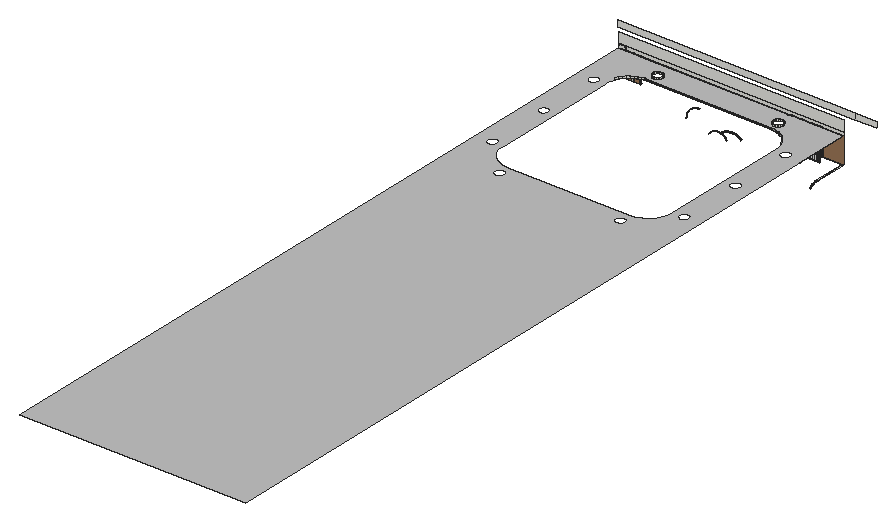
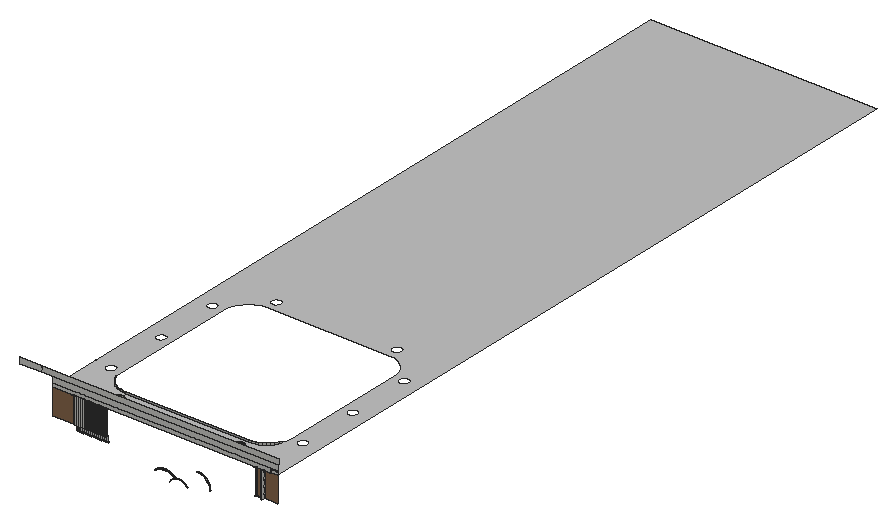
# SketchUp Ruby script. Lengths in inches.
U = 1.inch
M = Sketchup.active_model
def pt(a) = Geom::Point3d.new(a.map { |v| v * U })
def face(e, loops, mat)
  f = e.add_face(loops[0].map { |a| pt(a) })
  loops[1..].each { |l| e.add_face(l.map { |a| pt(a) }).erase! }
  f.material = f.back_material = mat if mat
  f
end
# faces: each face lists its corners as indices into pts; further lists are holes
def faces(e, pts, list, mat = nil) = list.each { |f| face(e, (f[0].is_a?(Array) ? f : [f]).map { |l| l.map { |i| pts[i] } }, mat) }
# xy, xz, yz: faces in a plane at the given z, y or x. An outline is a flat list of corners, or four numbers for a rectangle; further outlines are holes
def ring(l) = l.size == 4 ? [[l[0], l[1]], [l[2], l[1]], [l[2], l[3]], [l[0], l[3]]] : l.each_slice(2).to_a
def flat(e, list, mat, &to3) = list.each { |f| face(e, (f[0].is_a?(Array) ? f : [f]).map { |l| ring(l).map { |u, v| to3.(u, v) } }, mat) }
def xy(e, z, list, mat = nil) = flat(e, list, mat) { |x, y| [x, y, z] }
def xz(e, y, list, mat = nil) = flat(e, list, mat) { |x, z| [x, y, z] }
def yz(e, x, list, mat = nil) = flat(e, list, mat) { |y, z| [x, y, z] }
def lines(e, pts, list) = list.each { |a, b| e.add_line(pt(pts[a]), pt(pts[b])) }
# prism: a flat outline (further loops are holes) pulled along v
def prism(e, loops, v, mat = nil)
  f = face(e, loops, mat); d = Geom::Vector3d.new(v.map { |x| x * U })
  f.pushpull(f.normal.samedirection?(d) ? d.length : -d.length)
end
def box(e, o, s, mat = nil) = prism(e, [[o, [o[0] + s[0], o[1], o[2]], [o[0] + s[0], o[1] + s[1], o[2]], [o[0], o[1] + s[1], o[2]]]], [0, 0, s[2]], mat)
def at(x, y, z, deg = 0) = Geom::Transformation.translation(pt([x, y, z])) * Geom::Transformation.rotation(ORIGIN, Z_AXIS, deg.degrees)
def axes(o, x, y, z) = Geom::Transformation.new([*x, 0, *y, 0, *z, 0, *pt(o).to_a, 1])
def part(name) = M.definitions.add(name)
# library, detail: a bought-in or finely detailed component or shape, given as its bounding box
def library(name, o, s) = part(name).tap { |d| box(d.entities, o, s) }
def detail(e, o, s) = box(e.add_group.entities, o, s)
def put(e, d, t, mat = nil) = e.add_instance(d, t).tap { |i| i.material = mat if mat }
def group(e, t, mat = nil) = e.add_group.tap { |g| g.transformation = t; g.material = mat if mat }.entities
root = M.entities
M.materials.add("[0130_Gainsboro]").color = [220, 220, 220]
M.materials.add("[0131_Silver]1").color = [192, 192, 192]
M.materials.add("[Color D06]").color = [204, 153, 0]
M.materials.add("[Color M08]").color = [30, 30, 30]
M.materials.add("[Polished Concrete New]").color = [200, 200, 203]
M.materials.add("[Wood Floor]").color = [153, 117, 86]
xy(root,120.567,[[180.702,755.5,181.219,755.9375],[182.702,755.5,183.219,755.9375],[184.702,755.5,185.219,755.9375],[186.702,755.5,187.219,755.9375],[188.702,755.5,189.219,755.9375],
  [190.702,755.5,191.219,755.9375],[192.702,755.5,193.219,755.9375],[194.702,755.5,195.219,755.9375],[196.702,755.5,197.219,755.9375],[198.702,755.5,199.219,755.9375],
  [200.702,755.5,201.219,755.875],[202.702,755.5,203.219,755.875],[204.702,755.5,205.219,755.875],[206.702,755.5,207.219,755.875],[208.702,755.5,209.219,755.875]])
xy(root,121.254,[[180.702,755.5,181.219,755.9375],[182.702,755.5,183.219,755.9375],[184.702,755.5,185.219,755.9375],[186.702,755.5,187.219,755.9375],[188.702,755.5,189.219,755.9375],
  [190.702,755.5,191.219,755.9375],[192.702,755.5,193.219,755.9375],[194.702,755.5,195.219,755.9375],[196.702,755.5,197.219,755.9375],[198.702,755.5,199.219,755.9375],
  [200.702,755.5,201.219,755.875],[202.702,755.5,203.219,755.875],[204.702,755.5,205.219,755.875],[206.702,755.5,207.219,755.875],[208.702,755.5,209.219,755.875]])
xy(root,126.029,[[232.4375,723.825,233.031,755.5],[233.625,723.825,234,755.5],[212.702,755.5,233.625,756.094],[233.625,755.5,234,757.0625]])
xy(root,126.503,[[20.995,756.6875,27.258,756.6875,27.258,757.375,28.492,757.375,28.492,758.4375,20.995,757.25],[19.81,757.0625,19.81,758.0625,20.995,758.0625,20.995,757.25],[19.81,757.0625,20.995,757.25,20.995,757.0625],[19.81,758.0625,20.995,759.4375]])
xy(root,152.123,[[233.625,700.967,234,757.0625],[13.149,756.6875,19.81,757.0625],[20.995,756.6875,27.258,757.0625],[28.492,756.6875,179.219,757.0625],[212.702,756.6875,233.625,757.0625],
  [19.81,757.0625,20.995,758.0625],[27.258,757.0625,28.492,757.375],[180.702,757.0625,181.219,757.375],[182.702,757.0625,183.219,757.375],[184.702,757.0625,185.219,757.375],
  [186.702,757.0625,187.219,757.375],[188.702,757.0625,189.219,757.375],[190.702,757.0625,191.219,757.375],[192.702,757.0625,193.219,757.375],[194.702,757.0625,195.219,757.375],
  [196.702,757.0625,197.219,757.375],[198.702,757.0625,199.219,757.375],[200.702,757.0625,201.219,757.375],[202.702,757.0625,203.219,757.375],[204.702,757.0625,205.219,757.375],
  [206.702,757.0625,207.219,757.375],[208.702,757.0625,209.219,757.375],[210.702,757.0625,211.219,757.375],[19.81,758.0625,20.995,759.4375]])
xy(root,152.123,[[[6.399,0,6.399,756.6875,19.81,756.6875,19.81,757.0625,20.995,757.0625,20.995,756.6875,27.258,756.6875,27.258,757.0625,28.492,757.0625,28.492,756.6875,179.219,756.6875,179.219,757.0625,212.702,757.0625,212.702,756.6875,233.625,756.6875,233.625,700.967,234,700.967,234,0],[57.936,550.998,182.064,550.998,185.197,551.204,188.276,551.816,191.248,552.825,194.064,554.214,196.674,555.958,199.035,558.028,201.105,560.388,202.849,562.998,204.237,565.814,205.246,568.787,205.859,571.866,206.064,574.998,206.064,705.127,205.859,708.259,205.246,711.338,204.237,714.311,202.849,717.127,201.105,719.737,199.035,722.097,196.674,724.167,194.064,725.911,191.248,727.3,188.276,728.309,185.197,728.921,182.064,729.127,57.936,729.127,54.803,728.921,51.724,728.309,48.752,727.3,45.936,725.911,43.326,724.167,40.965,722.097,38.895,719.737,37.151,717.127,35.763,714.311,34.754,711.338,34.141,708.259,33.936,705.127,33.936,574.998,34.141,571.866,34.754,568.787,35.763,565.814,37.151,562.998,38.895,560.388,40.965,558.028,43.326,555.958,45.936,554.214,48.752,552.825,51.724,551.816,54.803,551.204],[217,635.915,218.294,636.085,219.5,636.585,220.536,637.379,221.33,638.415,221.83,639.621,222,640.915,221.83,642.209,221.33,643.415,220.536,644.45,219.5,645.245,218.294,645.744,217,645.915,215.706,645.744,214.5,645.245,213.464,644.45,212.67,643.415,212.17,642.209,212,640.915,212.17,639.621,212.67,638.415,213.464,637.379,214.5,636.585,215.706,636.085],[23,635.915,24.294,636.085,25.5,636.585,26.536,637.379,27.33,638.415,27.83,639.621,28,640.915,27.83,642.209,27.33,643.415,26.536,644.45,25.5,645.245,24.294,645.744,23,645.915,21.706,645.744,20.5,645.245,19.464,644.45,18.67,643.415,18.17,642.209,18,640.915,18.17,639.621,18.67,638.415,19.464,637.379,20.5,636.585,21.706,636.085],[217,571.0625,218.294,571.233,219.5,571.732,220.536,572.527,221.33,573.5625,221.83,574.768,222,576.0625,221.83,577.357,221.33,578.5625,220.536,579.598,219.5,580.393,218.294,580.892,217,581.0625,215.706,580.892,214.5,580.393,213.464,579.598,212.67,578.5625,212.17,577.357,212,576.0625,212.17,574.768,212.67,573.5625,213.464,572.527,214.5,571.732,215.706,571.233],[59,535.0625,60.294,535.233,61.5,535.732,62.536,536.527,63.33,537.5625,63.83,538.768,64,540.0625,63.83,541.357,63.33,542.5625,62.536,543.598,61.5,544.393,60.294,544.892,59,545.0625,57.706,544.892,56.5,544.393,55.464,543.598,54.67,542.5625,54.17,541.357,54,540.0625,54.17,538.768,54.67,537.5625,55.464,536.527,56.5,535.732,57.706,535.233],[181,535.0625,182.294,535.233,183.5,535.732,184.536,536.527,185.33,537.5625,185.83,538.768,186,540.0625,185.83,541.357,185.33,542.5625,184.536,543.598,183.5,544.393,182.294,544.892,181,545.0625,179.706,544.892,178.5,544.393,177.464,543.598,176.67,542.5625,176.17,541.357,176,540.0625,176.17,538.768,176.67,537.5625,177.464,536.527,178.5,535.732,179.706,535.233],[23,571.0625,24.294,571.233,25.5,571.732,26.536,572.527,27.33,573.5625,27.83,574.768,28,576.0625,27.83,577.357,27.33,578.5625,26.536,579.598,25.5,580.393,24.294,580.892,23,581.0625,21.706,580.892,20.5,580.393,19.464,579.598,18.67,578.5625,18.17,577.357,18,576.0625,18.17,574.768,18.67,573.5625,19.464,572.527,20.5,571.732,21.706,571.233],[23,699.0625,24.294,699.233,25.5,699.732,26.536,700.527,27.33,701.5625,27.83,702.768,28,704.0625,27.83,705.357,27.33,706.5625,26.536,707.598,25.5,708.393,24.294,708.892,23,709.0625,21.706,708.892,20.5,708.393,19.464,707.598,18.67,706.5625,18.17,705.357,18,704.0625,18.17,702.768,18.67,701.5625,19.464,700.527,20.5,699.732,21.706,699.233],[181,735.0625,182.294,735.233,183.5,735.732,184.536,736.527,185.33,737.5625,185.83,738.768,186,740.0625,185.83,741.357,185.33,742.5625,184.536,743.598,183.5,744.393,182.294,744.892,181,745.0625,179.706,744.892,178.5,744.393,177.464,743.598,176.67,742.5625,176.17,741.357,176,740.0625,176.17,738.768,176.67,737.5625,177.464,736.527,178.5,735.732,179.706,735.233],[59,735.0625,60.294,735.233,61.5,735.732,62.536,736.527,63.33,737.5625,63.83,738.768,64,740.0625,63.83,741.357,63.33,742.5625,62.536,743.598,61.5,744.393,60.294,744.892,59,745.0625,57.706,744.892,56.5,744.393,55.464,743.598,54.67,742.5625,54.17,741.357,54,740.0625,54.17,738.768,54.67,737.5625,55.464,736.527,56.5,735.732,57.706,735.233],[217,699.0625,218.294,699.233,219.5,699.732,220.536,700.527,221.33,701.5625,221.83,702.768,222,704.0625,221.83,705.357,221.33,706.5625,220.536,707.598,219.5,708.393,218.294,708.892,217,709.0625,215.706,708.892,214.5,708.393,213.464,707.598,212.67,706.5625,212.17,705.357,212,704.0625,212.17,702.768,212.67,701.5625,213.464,700.527,214.5,699.732,215.706,699.233]]],"[0131_Silver]1")
xy(root,155.498,[[6,756.6875,13.149,757.0625]])
xz(root,729.127,[[57.936,152.123,182.064,153.654]],"[0131_Silver]1")
xz(root,755.5,[[178.264,120.567,210.702,121.254],[179.219,121.254,180.702,126.029],[181.219,121.254,182.702,126.029],[183.219,121.254,184.702,126.029],[185.219,121.254,186.702,126.029],
  [187.219,121.254,188.702,126.029],[189.219,121.254,190.702,126.029],[191.219,121.254,192.702,126.029],[193.219,121.254,194.702,126.029],[195.219,121.254,196.702,126.029],
  [197.219,121.254,198.702,126.029],[199.219,121.254,200.702,126.029],[201.219,121.254,202.702,126.029],[203.219,121.254,204.702,126.029],[205.219,121.254,206.702,126.029],
  [207.219,121.254,208.702,126.029],[209.219,121.254,210.702,126.029]],"[0130_Gainsboro]")
xz(root,755.5,[[111.282,111.566,112.321,112.492,113.569,113.389,114.904,114.152,116.311,114.77,117.776,115.238,119.281,115.551,120.811,115.704,122.348,115.696,123.876,115.528,125.378,115.201,126.838,114.719,128.24,114.087,129.567,113.312,130.187,112.857,130.527,113.321,129.883,113.794,128.504,114.599,127.047,115.256,125.53,115.757,123.969,116.097,122.381,116.272,120.783,116.279,119.193,116.12,117.629,115.795,116.107,115.309,114.645,114.666,113.257,113.874,111.96,112.941,110.768,111.878,110.691,111.793],[110.691,111.793,110.768,111.878,111.96,112.941,113.257,113.874,114.645,114.666,116.107,115.309,117.629,115.795,119.193,116.12,120.783,116.279,122.381,116.272,123.969,116.097,125.53,115.757,127.047,115.256,128.504,114.599,129.883,113.794,130.527,113.321,130.745,113.618,130.085,114.102,128.672,114.927,127.181,115.599,125.627,116.112,124.028,116.46,122.402,116.639,120.766,116.647,119.138,116.484,117.536,116.151,115.977,115.653,114.479,114.995,113.058,114.184,111.73,113.228,110.509,112.14,110.291,111.9,110.688,111.794],[130.807,112.402,131.171,112.848,130.527,113.321,130.187,112.857],[131.171,112.848,131.404,113.133,131.404,113.134,130.745,113.618,130.527,113.321]],"[Color M08]")
xz(root,755.875,[[200.702,120.567,201.219,121.254],[202.702,120.567,203.219,121.254],[204.702,120.567,205.219,121.254],[206.702,120.567,207.219,121.254],[208.702,120.567,209.219,121.254]])
xz(root,755.9375,[[180.702,120.567,181.219,121.254],[182.702,120.567,183.219,121.254],[184.702,120.567,185.219,121.254],[186.702,120.567,187.219,121.254],[188.702,120.567,189.219,121.254],
  [190.702,120.567,191.219,121.254],[192.702,120.567,193.219,121.254],[194.702,120.567,195.219,121.254],[196.702,120.567,197.219,121.254],[198.702,120.567,199.219,121.254]])
xz(root,756.6875,[[6.399,152.123,13.149,155.498]])
xz(root,756.6875,[[212.702,126.029,233.625,152.123],[6,126.503,19.81,126.503,19.81,152.123,6.399,152.123,6.399,155.498,6,155.498],[20.995,126.503,27.258,152.123]],"[Wood Floor]")
xz(root,757.0625,[[13.149,152.123,13.149,155.498,6,155.498,6,156.123,234,156.123,234,152.123],[6,156.123,234,166.281]])
xz(root,757.0625,[[19.81,126.503,20.995,152.123]],"[Color D06]")
xz(root,757.0625,[[179.219,126.029,180.702,152.123],[181.219,126.029,182.702,152.123],[183.219,126.029,184.702,152.123],[185.219,126.029,186.702,152.123],[187.219,126.029,188.702,152.123],
  [189.219,126.029,190.702,152.123],[191.219,126.029,192.702,152.123],[193.219,126.029,194.702,152.123],[195.219,126.029,196.702,152.123],[197.219,126.029,198.702,152.123],
  [199.219,126.029,200.702,152.123],[201.219,126.029,202.702,152.123],[203.219,126.029,204.702,152.123],[205.219,126.029,206.702,152.123],[207.219,126.029,208.702,152.123],
  [209.219,126.029,210.702,152.123],[211.219,126.029,212.702,152.123]],"[Wood Floor]")
xz(root,757.375,[[27.258,126.503,28.492,152.123]],"[Color D06]")
xz(root,757.375,[[180.702,126.029,181.219,152.123],[182.702,126.029,183.219,152.123],[184.702,126.029,185.219,152.123],[186.702,126.029,187.219,152.123],[188.702,126.029,189.219,152.123],
  [190.702,126.029,191.219,152.123],[192.702,126.029,193.219,152.123],[194.702,126.029,195.219,152.123],[196.702,126.029,197.219,152.123],[198.702,126.029,199.219,152.123],
  [200.702,126.029,201.219,152.123],[202.702,126.029,203.219,152.123],[204.702,126.029,205.219,152.123],[206.702,126.029,207.219,152.123],[208.702,126.029,209.219,152.123],
  [210.702,126.029,211.219,152.123]],"[Wood Floor]")
xz(root,758.0625,[[19.81,126.503,20.995,152.123]])
xz(root,759.4375,[[19.81,126.503,20.995,152.123]])
xz(root,763.0625,[[0,166.281,240,172.281],[240,166.281,261.625,172.281]])
yz(root,13.149,[[756.6875,152.123,757.0625,155.498]])
yz(root,19.81,[[756.6875,126.503,757.0625,152.123],[757.0625,126.503,758.0625,152.123],[758.0625,126.503,759.4375,152.123]])
yz(root,20.995,[[756.6875,126.503,757.0625,152.123],[757.0625,126.503,758.0625,152.123],[758.0625,126.503,759.4375,152.123]])
yz(root,27.258,[[756.6875,126.503,757.375,152.123]])
yz(root,28.492,[[756.6875,126.503,757.375,152.123]])
yz(root,179.219,[[756.6875,126.029,757.0625,152.123]],"[Wood Floor]")
yz(root,180.702,[[757.0625,126.029,757.375,152.123]])
yz(root,181.219,[[757.0625,126.029,757.375,152.123]])
yz(root,182.702,[[757.0625,126.029,757.375,152.123]])
yz(root,183.219,[[757.0625,126.029,757.375,152.123]])
yz(root,184.702,[[757.0625,126.029,757.375,152.123]])
yz(root,185.219,[[757.0625,126.029,757.375,152.123]])
yz(root,186.702,[[757.0625,126.029,757.375,152.123]])
yz(root,187.219,[[757.0625,126.029,757.375,152.123]])
yz(root,188.702,[[757.0625,126.029,757.375,152.123]])
yz(root,189.219,[[757.0625,126.029,757.375,152.123]])
yz(root,190.702,[[757.0625,126.029,757.375,152.123]])
yz(root,191.219,[[757.0625,126.029,757.375,152.123]])
yz(root,192.702,[[757.0625,126.029,757.375,152.123]])
yz(root,193.219,[[757.0625,126.029,757.375,152.123]])
yz(root,194.702,[[757.0625,126.029,757.375,152.123]])
yz(root,195.219,[[757.0625,126.029,757.375,152.123]])
yz(root,196.702,[[757.0625,126.029,757.375,152.123]])
yz(root,197.219,[[757.0625,126.029,757.375,152.123]])
yz(root,198.702,[[757.0625,126.029,757.375,152.123]])
yz(root,199.219,[[757.0625,126.029,757.375,152.123]])
yz(root,200.702,[[757.0625,126.029,757.375,152.123]])
yz(root,201.219,[[757.0625,126.029,757.375,152.123]])
yz(root,202.702,[[757.0625,126.029,757.375,152.123]])
yz(root,203.219,[[757.0625,126.029,757.375,152.123]])
yz(root,204.702,[[757.0625,126.029,757.375,152.123]])
yz(root,205.219,[[757.0625,126.029,757.375,152.123]])
yz(root,206.702,[[757.0625,126.029,757.375,152.123]])
yz(root,207.219,[[757.0625,126.029,757.375,152.123]])
yz(root,208.702,[[755.8125,120.567,755.875,121.254],[755.5,121.254,755.8125,126.029],[757.0625,126.029,757.375,152.123]])
yz(root,209.219,[[755.8125,120.567,755.875,121.254],[755.5,121.254,755.8125,126.029],[757.0625,126.029,757.375,152.123]])
yz(root,210.702,[[757.0625,126.029,757.375,152.123]])
yz(root,211.219,[[757.0625,126.029,757.375,152.123]])
yz(root,212.702,[[756.6875,126.029,757.0625,152.123]])
p = [[99.337,755.5,108.106],[98.758,755.5,107.215],[98.758,755.246,107.215],[99.337,755.246,108.106],[116.343,755.5,107.215],[115.764,755.5,108.106],
  [115.764,755.246,108.106],[116.343,755.246,107.215],[100.005,755.5,108.932],[100.005,755.246,108.932],[115.192,755.5,108.8125],[115.096,755.5,108.932],
  [115.096,755.246,108.932],[100.757,755.5,109.683],[100.757,755.246,109.683],[114.621,755.5,109.407],[114.344,755.5,109.683],[114.344,755.246,109.683],
  [101.583,755.5,110.352],[101.583,755.246,110.352],[113.518,755.5,110.352],[113.518,755.246,110.352],[102.474,755.5,110.931],[102.474,755.246,110.931],
  [112.627,755.5,110.931],[112.627,755.246,110.931],[103.421,755.5,111.413],[103.421,755.246,111.413],[111.68,755.5,111.413],[111.68,755.246,111.413],
  [104.413,755.5,111.794],[104.413,755.246,111.794],[110.691,755.5,111.793],[110.688,755.5,111.794],[110.688,755.246,111.794],[111.282,755.5,111.566],
  [105.44,755.5,112.069],[105.44,755.246,112.069],[110.291,755.5,111.9],[109.661,755.5,112.069],[109.661,755.246,112.069],[106.489,755.5,112.235],
  [106.489,755.246,112.235],[108.612,755.5,112.235],[108.612,755.246,112.235],[107.551,755.5,112.291],[107.551,755.246,112.291],[75.568,755.5,114.727],
  [75.568,756.094,114.727],[75.457,756.094,113.03],[75.457,755.5,113.03],[75.9,755.5,116.395],[75.9,756.094,116.395],[76.447,755.5,118.005],
  [76.447,756.094,118.005],[77.199,755.5,119.53],[77.199,756.094,119.53],[78.143,755.5,120.944],[78.143,756.094,120.944],[79.264,755.5,122.222],
  [79.264,756.094,122.222],[80.543,755.5,123.343],[80.543,756.094,123.343],[232.4375,714.991,123.031],[233.031,714.991,123.031],[233.031,716.569,124.085],
  [232.4375,716.569,124.085],[234,714.991,123.031],[234,716.569,124.085],[233.625,716.569,124.085],[233.625,714.991,123.031],[81.957,755.5,124.288],
  [81.957,756.094,124.288],[233.031,718.272,124.925],[232.4375,718.272,124.925],[234,718.272,124.925],[233.625,718.272,124.925],[83.482,755.5,125.04],
  [83.482,756.094,125.04],[233.031,720.069,125.535],[232.4375,720.069,125.535],[234,720.069,125.535],[233.625,720.069,125.535],[85.092,755.5,125.586],
  [85.092,756.094,125.586],[233.031,721.931,125.905],[232.4375,721.931,125.905],[234,721.931,125.905],[233.625,721.931,125.905],[86.759,755.5,125.918],
  [86.759,756.094,125.918],[233.031,723.825,126.029],[232.4375,723.825,126.029],[234,723.825,126.029],[233.625,723.825,126.029],[88.456,755.5,126.029],
  [88.456,756.094,126.029],[37.151,717.127,152.123],[37.151,717.127,153.654],[35.763,714.311,153.654],[35.763,714.311,152.123],[204.237,714.311,152.123],
  [204.237,714.311,153.654],[202.849,717.127,153.654],[202.849,717.127,152.123],[38.895,719.737,152.123],[38.895,719.737,153.654],[201.105,719.737,153.654],
  [201.105,719.737,152.123],[40.965,722.097,152.123],[40.965,722.097,153.654],[199.035,722.097,153.654],[199.035,722.097,152.123],[43.326,724.167,152.123],
  [43.326,724.167,153.654],[196.674,724.167,153.654],[196.674,724.167,152.123],[45.936,725.911,152.123],[45.936,725.911,153.654],[194.064,725.911,153.654],
  [194.064,725.911,152.123],[48.752,727.3,152.123],[48.752,727.3,153.654],[191.248,727.3,153.654],[191.248,727.3,152.123],[51.724,728.309,152.123],
  [51.724,728.309,153.654],[188.276,728.309,153.654],[188.276,728.309,152.123],[54.803,728.921,152.123],[54.803,728.921,153.654],[185.197,728.921,153.654],
  [185.197,728.921,152.123],[57.936,729.127,152.123],[57.936,729.127,153.654],[182.064,729.127,153.654],[182.064,729.127,152.123],[59,735.0625,152.123],
  [57.706,735.233,152.123],[57.706,735.233,153.435],[59,735.0625,153.435],[60.294,735.233,152.123],[60.294,735.233,153.435],[181,735.0625,152.123],
  [179.706,735.233,152.123],[179.706,735.233,153.31],[181,735.0625,153.31],[182.294,735.233,152.123],[182.294,735.233,153.31],[56.5,735.732,152.123],
  [56.5,735.732,153.435],[61.5,735.732,152.123],[61.5,735.732,153.435],[178.5,735.732,152.123],[178.5,735.732,153.31],[183.5,735.732,152.123],
  [183.5,735.732,153.31],[55.464,736.527,152.123],[55.464,736.527,153.435],[62.536,736.527,152.123],[62.536,736.527,153.435],[177.464,736.527,152.123],
  [177.464,736.527,153.31],[184.536,736.527,152.123],[184.536,736.527,153.31],[54.67,737.5625,152.123],[54.67,737.5625,153.435],[63.33,737.5625,152.123],
  [63.33,737.5625,153.435],[176.67,737.5625,152.123],[176.67,737.5625,153.31],[185.33,737.5625,152.123],[185.33,737.5625,153.31],[54.17,738.768,152.123],
  [54.17,738.768,153.435],[63.83,738.768,152.123],[63.83,738.768,153.435],[176.17,738.768,152.123],[176.17,738.768,153.31],[185.83,738.768,152.123],
  [185.83,738.768,153.31],[54,740.0625,152.123],[54,740.0625,153.435],[64,740.0625,152.123],[64,740.0625,153.435],[176,740.0625,152.123],
  [176,740.0625,153.31],[186,740.0625,152.123],[186,740.0625,153.31],[54.17,741.357,152.123],[54.17,741.357,153.435],[63.83,741.357,152.123],
  [63.83,741.357,153.435],[176.17,741.357,152.123],[176.17,741.357,153.31],[185.83,741.357,152.123],[185.83,741.357,153.31],[54.67,742.5625,152.123],
  [54.67,742.5625,153.435],[63.33,742.5625,152.123],[63.33,742.5625,153.435],[176.67,742.5625,152.123],[176.67,742.5625,153.31],[185.33,742.5625,152.123],
  [185.33,742.5625,153.31],[55.464,743.598,152.123],[55.464,743.598,153.435],[62.536,743.598,152.123],[62.536,743.598,153.435],[177.464,743.598,152.123],
  [177.464,743.598,153.31],[184.536,743.598,152.123],[184.536,743.598,153.31],[56.5,744.393,152.123],[56.5,744.393,153.435],[61.5,744.393,152.123],
  [61.5,744.393,153.435],[178.5,744.393,152.123],[178.5,744.393,153.31],[183.5,744.393,152.123],[183.5,744.393,153.31],[57.706,744.892,152.123],
  [57.706,744.892,153.435],[60.294,744.892,152.123],[60.294,744.892,153.435],[179.706,744.892,152.123],[179.706,744.892,153.31],[182.294,744.892,152.123],
  [182.294,744.892,153.31],[59,745.0625,152.123],[59,745.0625,153.435],[181,745.0625,152.123],[181,745.0625,153.31],[192.702,757.375,126.029],
  [192.702,757.5625,126.029]]
faces(root,p,[[0,1,2,3],[4,5,6,7],[8,0,3,9],[10,11,12,6,5],[13,8,9,14],[15,16,17,12,11],[18,13,14,19],[16,20,21,17],
  [22,18,19,23],[20,24,25,21],[26,22,23,27],[24,28,29,25],[30,26,27,31],[32,33,34,29,28,35],[36,30,31,37],[38,39,40,34,33],
  [41,36,37,42],[39,43,44,40],[45,41,42,46],[43,45,46,44],[47,48,49,50],[51,52,48,47],[53,54,52,51],[55,56,54,53],
  [57,58,56,55],[59,60,58,57],[61,62,60,59],[67,68,69,70],[71,72,62,61],[68,75,76,69],[77,78,72,71],[75,81,82,76],
  [83,84,78,77],[81,87,88,82],[89,90,84,83],[87,93,94,88],[95,96,90,89],[97,98,99,100],[105,106,98,97],[109,110,106,105],
  [113,114,110,109],[117,118,114,113],[121,122,118,117],[125,126,122,121],[129,130,126,125],[133,134,130,129],[137,138,139,140],[141,137,140,142],
  [143,144,145,146],[147,143,146,148],[138,149,150,139],[151,141,142,152],[144,153,154,145],[155,147,148,156],[149,157,158,150],[159,151,152,160],
  [153,161,162,154],[163,155,156,164],[157,165,166,158],[167,159,160,168],[161,169,170,162],[171,163,164,172],[165,173,174,166],[175,167,168,176],
  [169,177,178,170],[179,171,172,180],[173,181,182,174],[183,175,176,184],[177,185,186,178],[187,179,180,188],[181,189,190,182],[191,183,184,192],
  [185,193,194,186],[195,187,188,196],[189,197,198,190],[199,191,192,200],[193,201,202,194],[203,195,196,204],[197,205,206,198],[207,199,200,208],
  [201,209,210,202],[211,203,204,212],[205,213,214,206],[215,207,208,216],[209,217,218,210],[219,211,212,220],[213,221,222,214],[223,215,216,224],
  [217,225,226,218],[227,219,220,228],[221,229,230,222],[229,223,224,230],[225,231,232,226],[231,227,228,232]])
faces(root,p,[[63,64,65,66],[66,65,73,74],[74,73,79,80],[80,79,85,86],[86,85,91,92]],"[Polished Concrete New]")
faces(root,p,[[101,102,103,104],[104,103,107,108],[108,107,111,112],[112,111,115,116],[116,115,119,120],[120,119,123,124],[124,123,127,128],[128,127,131,132],
  [132,131,135,136]],"[0131_Silver]1")
lines(root,p,[[233,234]])
